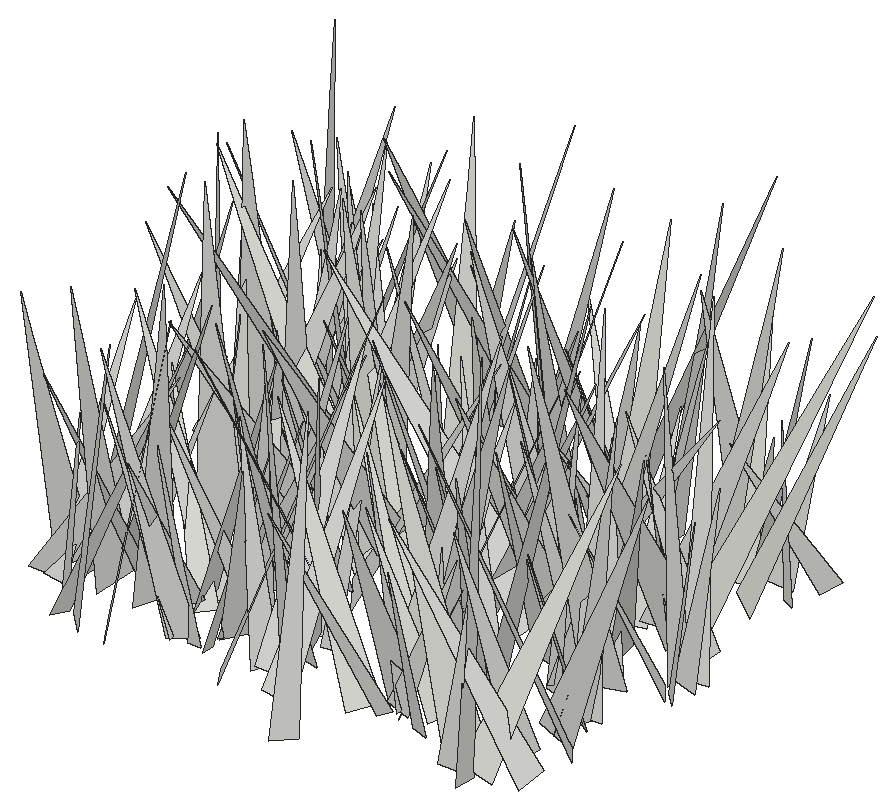
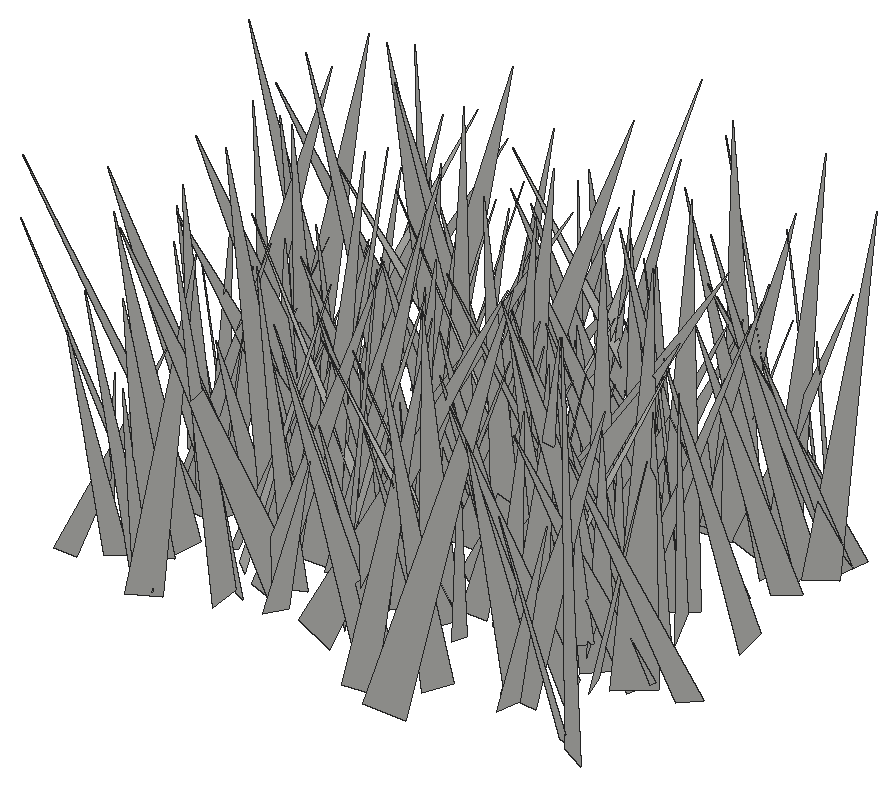
# SketchUp Ruby script. Lengths in inches.
U = 1.inch
M = Sketchup.active_model
def pt(a) = Geom::Point3d.new(a.map { |v| v * U })
def face(e, loops, mat)
  f = e.add_face(loops[0].map { |a| pt(a) })
  loops[1..].each { |l| e.add_face(l.map { |a| pt(a) }).erase! }
  f.material = f.back_material = mat if mat
  f
end
# faces: each face lists its corners as indices into pts; further lists are holes
def faces(e, pts, list, mat = nil) = list.each { |f| face(e, (f[0].is_a?(Array) ? f : [f]).map { |l| l.map { |i| pts[i] } }, mat) }
# xy, xz, yz: faces in a plane at the given z, y or x. An outline is a flat list of corners, or four numbers for a rectangle; further outlines are holes
def ring(l) = l.size == 4 ? [[l[0], l[1]], [l[2], l[1]], [l[2], l[3]], [l[0], l[3]]] : l.each_slice(2).to_a
def flat(e, list, mat, &to3) = list.each { |f| face(e, (f[0].is_a?(Array) ? f : [f]).map { |l| ring(l).map { |u, v| to3.(u, v) } }, mat) }
def xy(e, z, list, mat = nil) = flat(e, list, mat) { |x, y| [x, y, z] }
def xz(e, y, list, mat = nil) = flat(e, list, mat) { |x, z| [x, y, z] }
def yz(e, x, list, mat = nil) = flat(e, list, mat) { |y, z| [x, y, z] }
def lines(e, pts, list) = list.each { |a, b| e.add_line(pt(pts[a]), pt(pts[b])) }
# prism: a flat outline (further loops are holes) pulled along v
def prism(e, loops, v, mat = nil)
  f = face(e, loops, mat); d = Geom::Vector3d.new(v.map { |x| x * U })
  f.pushpull(f.normal.samedirection?(d) ? d.length : -d.length)
end
def box(e, o, s, mat = nil) = prism(e, [[o, [o[0] + s[0], o[1], o[2]], [o[0] + s[0], o[1] + s[1], o[2]], [o[0], o[1] + s[1], o[2]]]], [0, 0, s[2]], mat)
def at(x, y, z, deg = 0) = Geom::Transformation.translation(pt([x, y, z])) * Geom::Transformation.rotation(ORIGIN, Z_AXIS, deg.degrees)
def axes(o, x, y, z) = Geom::Transformation.new([*x, 0, *y, 0, *z, 0, *pt(o).to_a, 1])
def part(name) = M.definitions.add(name)
# library, detail: a bought-in or finely detailed component or shape, given as its bounding box
def library(name, o, s) = part(name).tap { |d| box(d.entities, o, s) }
def detail(e, o, s) = box(e.add_group.entities, o, s)
def put(e, d, t, mat = nil) = e.add_instance(d, t).tap { |i| i.material = mat if mat }
def group(e, t, mat = nil) = e.add_group.tap { |g| g.transformation = t; g.material = mat if mat }.entities
root = M.entities
c1 = part("fur_instance\#9")
p = [[0.8125,0,1.79],[0.67,-0.02,1.48],[0,-0.11,0],[0,0.11,0]]
faces(c1.entities,p,[[0,1,2,3]])
put(root,c1,axes([150.06,394.9,-27.1],[-5.67085,1.89535,1.35099],[1.57668,5.74544,-1.44226],[1.71219,0.98676,5.80265]))
put(root,c1,axes([155.92,397,-27.1],[0.94774,-3.5048,1.15841],[-3.67796,-0.79512,0.60341],[0.31324,1.26803,3.58018]))
put(root,c1,axes([140.08,397.19,-27.1],[6.22111,3.48137,1.76986],[3.77865,-6.20685,-1.07301],[-0.98698,-1.81924,7.04775]))
put(root,c1,axes([158.84,398.09,-27.1],[-5.67147,0.82087,0.04901],[0.80443,5.46726,1.5178],[-0.17066,-1.50898,5.5259]))
put(root,c1,axes([138.85,396.97,-27.1],[4.00395,3.96639,1.91354],[4.25291,-4.1539,-0.28869],[-1.14309,-1.56151,5.62855]))
put(root,c1,axes([153.53,398.33,-27.1],[-0.97443,-3.66118,0.75209],[-3.71136,1.03977,0.25308],[0.44234,0.6588,3.78017]))
put(root,c1,axes([142.61,398.41,-27.1],[0.82361,-5.861,1.93807],[-5.93962,-1.28507,-1.3621],[-1.68178,1.66825,5.75972]))
put(root,c1,axes([151.41,400.09,-27.1],[5.27025,-2.47106,0.85487],[-2.00329,-5.05203,-2.25305],[-1.68041,-1.72721,5.36707]))
put(root,c1,axes([157.63,399.32,-27.1],[-4.78026,1.17069,2.19317],[1.89155,4.79719,1.56216],[1.61324,-2.15588,4.66702]))
put(root,c1,axes([155.46,398.49,-27.1],[3.76435,-5.16952,3.38659],[-5.24976,-4.76711,-1.44149],[-3.26082,1.70703,6.23028]))
put(root,c1,axes([137.65,397.86,-27.1],[-2.04031,-2.94511,1.87891],[-3.25881,2.38849,0.20512],[1.25863,1.41005,3.57693]))
put(root,c1,axes([138.14,400.1,-27.1],[6.98441,-2.34407,2.00985],[-1.86712,-7.16517,-1.86827],[-2.45928,-1.21733,7.12645]))
put(root,c1,axes([151.6875,398.65,-27.1],[-1.12844,-4.06047,0.83548],[-3.60524,0.5338,-2.27512],[-2.04639,1.29864,3.54749]))
put(root,c1,axes([141.48,400.43,-27.1],[3.03189,-3.59681,0.02756],[-3.43565,-2.90654,-1.37057],[-1.06494,-0.8632,4.50011]))
put(root,c1,axes([157.08,396.49,-27.1],[-7.37531,-1.40171,2.74866],[-2.16749,7.42249,-2.03071],[2.19589,2.61858,7.22747]))
put(root,c1,axes([143.98,399.68,-27.1],[3.85722,-2.97975,0.1804],[-2.96484,-3.85827,-0.33622],[-0.3481,-0.15623,4.86251]))
put(root,c1,axes([142.22,398.5,-27.1],[-4.50006,-1.01814,0.39176],[-1.03948,4.50642,-0.22865],[0.331,0.31016,4.60813]))
put(root,c1,axes([147.51,401.94,-27.1],[-4.65731,-6.85842,0.0184],[-6.74044,4.58127,1.51895],[1.26677,-0.83835,8.14992]))
put(root,c1,axes([136.05,400.48,-27.1],[5.91516,-3.3432,1.65321],[-2.9566,-6.09276,-1.74243],[-2.27346,-0.77492,6.56735]))
put(root,c1,axes([143.23,398.31,-27.1],[0.75971,3.71481,1.88794],[3.89435,-1.31575,1.02184],[-1.48263,-1.55251,3.65142]))
put(root,c1,axes([146.2,398.67,-27.1],[-4.24357,2.27798,1.78244],[2.54082,4.44811,0.36434],[1.38223,-1.18292,4.80254]))
put(root,c1,axes([140.07,399.95,-27.1],[6.97183,-3.45055,1.53762],[-3.37643,-7.13932,-0.71191],[-1.69419,0.0288,7.74635]))
put(root,c1,axes([148.16,397.59,-27.1],[-6.10428,-1.79449,1.71008],[-2.20054,6.01533,-1.54278],[1.14113,2.0006,6.1727]))
put(root,c1,axes([139.66,400.42,-27.1],[-1.20375,-5.21342,0.24756],[-5.17288,1.15789,-0.76855],[-0.69453,0.4118,5.2951]))
put(root,c1,axes([151.89,399.15,-27.1],[0.78956,-4.05986,1.16414],[-3.93825,-0.27989,1.69498],[1.52574,1.37851,3.77266]))
put(root,c1,axes([150.81,398.53,-27.1],[-4.45803,3.98436,0.74293],[4.03358,4.25341,1.39275],[-0.39655,-1.52789,5.81458]))
put(root,c1,axes([137.97,397.15,-27.1],[5.78446,0.51407,0.77192],[0.25637,-5.57234,1.78981],[-0.89129,1.73346,5.52457]))
put(root,c1,axes([147.09,399.9,-27.1],[-2.90211,-6.23156,1.67253],[-6.44447,2.71044,-1.08359],[-0.31368,1.96803,6.78825]))
put(root,c1,axes([156.99,397.26,-27.1],[0.07577,6.70614,0.84141],[6.48392,0.16538,-1.90197],[1.90764,-0.82847,6.43122]))
put(root,c1,axes([153.46,399.5625,-27.1],[-3.79672,1.89832,0.59417],[1.98792,3.66583,0.99077],[0.06937,-1.15319,4.1276]))
put(root,c1,axes([147.94,397.125,-27.1],[0.187,6.43803,0.46404],[6.40843,-0.12967,-0.78342],[0.77175,-0.48321,6.39292]))
put(root,c1,axes([135.7,399.11,-27.1],[4.06898,-3.86093,0.67624],[-3.71406,-3.48612,2.44405],[1.25293,2.20473,5.04877]))
put(root,c1,axes([158.81,400.48,-27.1],[-5.4011,-4.4458,0.12135],[-4.40164,5.31613,-1.14717],[-0.63674,0.96192,6.9008]))
put(root,c1,axes([143.81,398.35,-27.1],[3.84083,1.33111,0.88578],[1.09907,-3.87194,1.0529],[-1.16125,0.73803,3.92622]))
put(root,c1,axes([152,399.375,-27.1],[-4.7779,-0.84592,1.0787],[-0.97294,4.84801,-0.50762],[0.9657,0.69908,4.82558]))
put(root,c1,axes([145.41,397.03,-27.1],[6.47525,4.61232,0.40047],[4.47579,-6.41261,1.48613],[-1.18373,0.98374,7.80985]))
put(root,c1,axes([152.64,400.59,-27.1],[1.6475,-3.20979,0.84583],[-3.31321,-1.64761,0.20101],[-0.20196,0.8456,3.6023]))
put(root,c1,axes([157.54,401.13,-27.1],[1.03631,-6.95808,1.71035],[-6.57848,-0.23906,3.0134],[2.83968,1.98547,6.35675]))
put(root,c1,axes([146.55,401.06,-27.1],[5.52429,1.58059,2.16664],[1.98524,-5.74559,-0.8703],[-1.80317,-1.48335,5.67966]))
put(root,c1,axes([137.67,401.22,-27.1],[7.30646,0.41261,0.41525],[0.46932,-7.23653,-1.06747],[-0.34987,-1.09065,7.23983]))
put(root,c1,axes([143.98,401.01,-27.1],[-0.35504,-4.51922,1.36303],[-4.31721,-0.2418,-1.92625],[-1.90863,1.3876,4.10353]))
put(root,c1,axes([146.66,398.4375,-27.1],[-1.23708,6.4323,0.84499],[6.38548,1.35924,-0.99849],[1.14637,-0.62994,6.47363]))
put(root,c1,axes([141.63,400.9,-27.1],[5.98361,0.11352,0.76596],[0.13466,-6.02993,-0.15823],[-0.76252,-0.17402,5.9826]))
put(root,c1,axes([136.29,398.97,-27.1],[0.97806,5.36378,0.25201],[5.36787,-0.98334,0.09641],[-0.14015,-0.23057,5.45137]))
put(root,c1,axes([143.35,401.77,-27.1],[4.53528,-3.04969,1.17101],[-3.07507,-4.66168,-0.23091],[-1.10265,0.45689,5.46041]))
put(root,c1,axes([149.2,400.67,-27.1],[-4.27231,-1.94809,0.06255],[-1.87913,4.07681,-1.37844],[-0.51754,1.27912,4.48861]))
put(root,c1,axes([157.16,401.75,-27.1],[4.10425,1.09153,0.3293],[1.14011,-3.92312,-1.20584],[0.00571,-1.24998,4.07214]))
put(root,c1,axes([151.17,400.07,-27.1],[1.96643,7.28816,1.86053],[7.47956,-1.69089,-1.28167],[0.79683,-2.11408,7.43918]))
put(root,c1,axes([143.74,399.33,-27.1],[3.9731,1.20771,1.01378],[0.70264,-3.81635,1.79266],[-1.41159,1.49959,3.74573]))
put(root,c1,axes([151.63,400.76,-27.1],[-3.45745,4.3845,0.64107],[4.38114,3.2607,1.32749],[-0.66366,-1.31634,5.42361]))
put(root,c1,axes([152.15,403.32,-27.1],[-0.85203,-5.57664,0.61964],[-5.3803,0.98986,1.51043],[1.59225,0.36067,5.43539]))
put(root,c1,axes([150.91,402.38,-27.1],[6.79044,-4.4332,0.71146],[-4.48312,-6.76549,0.63187],[-0.24718,0.91888,8.0848]))
put(root,c1,axes([141.97,400.49,-27.1],[-2.66965,3.73747,0.14274],[3.69986,2.61324,0.77338],[-0.54785,-0.56423,4.52743]))
put(root,c1,axes([141.83,401.4,-27.1],[-5.56985,2.38046,0.65327],[2.45077,5.52546,0.76123],[0.29505,-0.95874,6.00918]))
put(root,c1,axes([152.17,399.02,-27.1],[5.76242,3.50846,0.12226],[3.39302,-5.62636,1.53663],[-0.90093,1.2508,6.56914]))
put(root,c1,axes([157.83,402.36,-27.1],[-2.17535,-3.01047,0.60266],[-3.06621,2.16789,-0.23847],[0.15643,0.62897,3.70651]))
put(root,c1,axes([152.35,403.72,-27.1],[-3.97091,-3.72473,0.66515],[-3.58252,4.01146,1.07602],[1.21718,-0.34456,5.33703]))
put(root,c1,axes([136.98,400.17,-27.1],[7.21368,2.51232,2.17903],[2.05011,-7.45745,1.81123],[-2.61859,1.08246,7.42081]))
put(root,c1,axes([146.46,401.7,-27.1],[-0.50007,3.75556,1.02909],[3.87876,0.38868,0.46638],[-0.34425,-1.07612,3.75989]))
put(root,c1,axes([147.2,406.47,-27.1],[4.97759,-6.71856,0.2944],[-6.18791,-4.7191,-3.07278],[-2.63353,-1.61035,7.77647]))
put(root,c1,axes([142.9,400.64,-27.1],[1.96135,3.70682,0.36248],[3.45553,-1.96392,1.38604],[-1.38968,0.34826,3.95807]))
put(root,c1,axes([149.18,404.94,-27.1],[7.15666,-2.1147,0.99823],[-1.83229,-7.06792,-1.83669],[-1.45298,-1.50292,7.233]))
put(root,c1,axes([157.6875,402.47,-27.1],[5.90361,-0.69248,2.28384],[-0.937,-6.27702,0.51884],[-2.19488,0.81708,5.9214]))
put(root,c1,axes([150.68,405.24,-27.1],[-1.15105,-5.30671,0.17],[-5.09537,1.15297,1.49093],[1.49242,-0.15644,5.22142]))
put(root,c1,axes([142.31,403.23,-27.1],[-3.28529,-1.60429,1.12724],[-1.66632,3.44368,0.04462],[1.03333,0.45264,3.6558]))
put(root,c1,axes([156.66,405.05,-27.1],[1.61042,-7.88282,1.5376],[-7.97737,-1.75156,-0.62458],[-0.92985,1.37466,8.02136]))
put(root,c1,axes([142.35,402.32,-27.1],[5.41003,-2.25588,0.78895],[-2.38957,-5.13634,1.69936],[-0.03699,1.87321,5.60977]))
put(root,c1,axes([136.34,402.07,-27.1],[-0.72846,5.64896,1.65026],[5.62241,1.15927,-1.48642],[1.73859,-1.38206,5.49837]))
put(root,c1,axes([153.78,405.26,-27.1],[-0.77388,-5.77446,0.46112],[-5.72229,0.83441,0.84559],[0.90132,0.33953,5.76439]))
put(root,c1,axes([153.49,402.61,-27.1],[8.05424,1.38868,1.7961],[1.29513,-8.24767,0.56905],[-1.86468,0.26973,8.15325]))
put(root,c1,axes([147.1875,401.08,-27.1],[1.91748,5.33638,0.31642],[5.10909,-1.9283,1.55969],[-1.57297,0.24194,5.4517]))
put(root,c1,axes([150.89,405,-27.1],[-5.52316,-3.7636,0.965],[-3.71814,5.60658,0.58551],[1.12752,0.05244,6.65787]))
put(root,c1,axes([137.57,402.83,-27.1],[2.54826,3.20038,0.28055],[3.20908,-2.5526,-0.02947],[-0.15164,-0.23787,4.09087]))
put(root,c1,axes([138.67,405.51,-27.1],[5.1556,-5.75467,2.21602],[-5.90961,-5.43588,-0.36737],[-1.76168,1.39363,7.71761]))
put(root,c1,axes([145.36,404.65,-27.1],[5.77692,4.11347,0.10405],[3.90568,-5.42514,-2.37018],[1.29504,-1.98782,6.68399]))
put(root,c1,axes([158.59,406.08,-27.1],[-3.47143,-2.84551,0.09651],[-2.81271,3.45107,0.57956],[0.4415,-0.38766,4.45106]))
put(root,c1,axes([155.74,407.03,-27.1],[6.93671,-0.62868,0.23505],[-0.51232,-6.5363,-2.3628],[-0.4336,-2.33453,6.55213]))
put(root,c1,axes([157.57,402.875,-27.1],[1.24745,7.40868,1.63783],[7.39275,-1.56046,1.42803],[-1.70827,-1.34297,7.376]))
put(root,c1,axes([155.36,405.58,-27.1],[0.47741,-4.86513,1.33169],[-4.92648,-0.73691,-0.92606],[-1.08291,1.20759,4.79999]))
put(root,c1,axes([144.97,404.88,-27.1],[0.7235,3.49331,2.20248],[3.65755,-1.58024,1.30491],[-1.91742,-1.69623,3.32022]))
put(root,c1,axes([142.81,403.1,-27.1],[5.29795,0.17393,1.896],[-0.4687,-5.31448,1.7972],[-1.84537,1.84915,4.98684]))
put(root,c1,axes([141.83,407.66,-27.1],[2.44843,-5.51273,0.60157],[-4.8536,-2.44839,-2.68234],[-2.6823,-0.60174,5.40279]))
put(root,c1,axes([138.97,404.72,-27.1],[5.52113,3.74347,2.2115],[4.00437,-5.77059,-0.2291],[-1.6939,-1.44011,6.66663]))
put(root,c1,axes([155.43,403.62,-27.1],[2.35955,4.93164,1.36493],[4.86886,-2.62618,1.07189],[-1.57426,-0.73054,5.36093]))
put(root,c1,axes([152.09,408.16,-27.1],[4.15216,-5.25606,0.30062],[-4.95254,-4.0295,-2.04756],[-1.78575,-1.04593,6.37763]))
put(root,c1,axes([151.65,404.47,-27.1],[-4.9618,2.41645,1.1014],[2.44275,5.06865,-0.11597],[1.04177,-0.37582,5.51772]))
put(root,c1,axes([149.36,404.625,-27.1],[-0.86303,4.80618,1.97762],[4.83833,1.47497,-1.47315],[1.8976,-1.57489,4.65553]))
put(root,c1,axes([155.25,405.69,-27.1],[-0.48209,-3.49328,1.24378],[-3.69826,0.54426,0.09516],[0.26993,1.21786,3.5251]))
put(root,c1,axes([157.15,409.34,-27.1],[4.52461,-6.7861,0.00105],[-6.53347,-4.35651,-2.20405],[-1.83437,-1.22185,7.85273]))
put(root,c1,axes([149.17,404.12,-27.1],[-2.13966,5.92839,0.3544],[5.56639,1.87053,2.31645],[-2.07043,-1.09766,5.86157]))
put(root,c1,axes([152.4375,408.11,-27.1],[-3.66849,-5.82093,1.22872],[-5.44278,3.86666,2.06783],[2.40191,-0.1285,6.56241]))
put(root,c1,axes([151.82,407.34,-27.1],[-7.78216,2.50032,0.23977],[2.4235,7.26917,2.85602],[-0.66011,-2.78901,7.65877]))
put(root,c1,axes([139.53,407.34,-27.1],[-6.5147,0.26004,1.16019],[0.55336,6.38259,1.67669],[1.05235,-1.74639,6.3006]))
put(root,c1,axes([156.18,405.84,-27.1],[-2.69115,3.5868,1.84623],[3.86426,2.92918,-0.05799],[1.15809,-1.43902,4.48375]))
put(root,c1,axes([159.03,405.85,-27.1],[-2.22453,-2.28888,1.93607],[-2.6411,2.63697,0.08289],[1.41842,1.32035,3.19071]))
put(root,c1,axes([144.74,407.35,-27.1],[4.88048,-6.02987,2.56967],[-6.14977,-5.32095,-0.80587],[-2.26779,1.4525,7.7155]))
put(root,c1,axes([158.85,406.87,-27.1],[0.22976,-4.49295,1.68417],[-4.67204,0.17468,1.10336],[1.09322,1.69077,4.36142]))
put(root,c1,axes([144.38,408.95,-27.1],[-2.23996,-8.03771,0.28468],[-7.44594,1.96073,-3.22749],[-3.04036,1.11981,7.69451]))
put(root,c1,axes([135.1,405.7,-27.1],[6.05583,0.88682,1.38397],[0.67013,-6.15634,1.01257],[-1.50092,0.82941,6.03608]))
put(root,c1,axes([155.43,404.32,-27.1],[7.73551,0.03019,2.73159],[-1.01366,-7.58581,2.95441],[-2.53672,3.12332,7.14916]))
put(root,c1,axes([144.4375,407.9,-27.1],[0.04247,-7.07988,2.41623],[-7.48051,-0.06275,-0.05238],[-0.06984,2.41579,7.07981]))
put(root,c1,axes([149.96,406.57,-27.1],[5.54197,-0.978,0.47716],[-1.05474,-5.437,1.10644],[-0.26776,1.17482,5.51777]))
put(root,c1,axes([139.78,408.5625,-27.1],[6.66168,-2.88093,2.18206],[-2.80757,-7.00677,-0.67958],[-2.27567,0.211,7.22605]))
put(root,c1,axes([158.44,407.0625,-27.1],[-5.81537,-0.03657,1.70774],[-0.23888,6.01751,-0.6846],[1.69135,0.72416,5.77505]))
put(root,c1,axes([145.93,408.32,-27.1],[-2.3451,-4.39084,0.71964],[-4.31416,2.04482,-1.58228],[-1.08875,1.35503,4.71968]))
put(root,c1,axes([144.76,406.84,-27.1],[-4.02573,7.19257,0.41274],[6.48293,3.4104,3.80141],[-3.14246,-2.17854,7.31361]))
put(root,c1,axes([157.27,408.23,-27.1],[-3.81411,-2.18756,1.38745],[-2.30966,3.98998,-0.05835],[1.17299,0.74331,4.39652]))
put(root,c1,axes([151.97,407.66,-27.1],[4.55,-4.60588,0.41001],[-4.16176,-3.82822,3.1795],[2.01545,2.49305,5.6398]))
put(root,c1,axes([142.47,405.12,-27.1],[2.76635,7.35948,0.05567],[7.35952,-2.76581,-0.07342],[0.04914,-0.07794,7.86188]))
put(root,c1,axes([143.23,409.17,-27.1],[0.67729,-7.55263,2.0847],[-7.70125,-0.25666,1.57216],[1.44182,2.17688,7.41817]))
put(root,c1,axes([158.24,408.97,-27.1],[-5.1344,0.67452,1.09766],[0.89094,5.11676,1.02317],[0.93062,-1.17714,5.07643]))
put(root,c1,axes([144.15,410.25,-27.1],[0.26999,-5.16111,0.17986],[-5.16087,-0.27616,-0.17741],[-0.18667,0.17024,5.16512]))
put(root,c1,axes([137.7,406.43,-27.1],[-6.50203,-1.48304,1.94789],[-2.15091,6.10063,-2.53495],[1.1693,2.97539,6.16846]))
put(root,c1,axes([138.15,407.15,-27.1],[0.38602,5.6901,1.15392],[5.67114,-0.61727,1.14668],[-1.24374,-1.04858,5.58671]))
put(root,c1,axes([137.91,409.85,-27.1],[3.24769,-2.54753,0.32293],[-2.51539,-3.26077,-0.4265],[-0.51676,-0.13836,4.10555]))
put(root,c1,axes([150.83,410.82,-27.1],[-0.69616,-7.71222,1.47846],[-7.81205,0.83092,0.65597],[0.79755,1.40715,7.71575]))
put(root,c1,axes([152.71,411.24,-27.1],[3.43107,-2.8474,0.0502],[-2.64084,-3.2106,-1.6126],[-1.06592,-1.21113,4.15686]))
put(root,c1,axes([138.87,407.95,-27.1],[-2.71022,2.78687,0.60598],[2.7235,2.77712,-0.59105],[0.8464,-0.01233,3.84222]))
put(root,c1,axes([153.89,411.8,-27.1],[-4.54437,-2.07997,0.71062],[-1.49312,4.11891,2.50752],[1.61302,-2.04715,4.32318]))
put(root,c1,axes([149.75,410.67,-27.1],[-6.14349,2.42883,3.06477],[3.31416,6.26335,1.67969],[2.07568,-2.81172,6.38908]))
put(root,c1,axes([151.89,409.95,-27.1],[4.55769,0.07164,0.01251],[0.0727,-4.46545,-0.91231],[0.00209,-0.91239,4.46602]))
put(root,c1,axes([158.87,407.35,-27.1],[0.5538,7.06628,1.29605],[7.05626,-0.7792,1.23321],[-1.34954,-1.17443,6.97985]))
put(root,c1,axes([148.31,408.86,-27.1],[4.95013,-1.23925,0.4471],[-1.29852,-4.88303,0.8422],[-0.22245,0.9272,5.03291]))
put(root,c1,axes([147.76,411.75,-27.1],[0.04578,-6.29285,0.19538],[-6.21134,-0.07706,-1.02644],[-1.02831,0.18529,6.20874]))
put(root,c1,axes([136.24,410.95,-27.1],[5.79688,-5.3049,1.7816],[-5.31494,-6.02201,-0.63769],[-1.75142,0.71643,7.83193]))
put(root,c1,axes([148.92,409.12,-27.1],[6.16739,3.42449,0.19717],[3.4017,-6.05394,-1.25736],[0.441,-1.19388,6.94138]))
put(root,c1,axes([148.3,408.59,-27.1],[2.54415,2.86578,1.34064],[2.68524,-2.86561,1.02977],[-1.67317,-0.2414,3.6912]))
put(root,c1,axes([147.15,409.23,-27.1],[-5.93557,-1.05009,0.32847],[-1.08922,5.86272,-0.94003],[0.15548,0.98355,5.95399]))
put(root,c1,axes([146.39,411.46,-27.1],[5.5268,-1.95543,1.04999],[-1.67194,-5.52102,-1.48142],[-1.45972,-1.07995,5.67227]))
put(root,c1,axes([137.53,408.62,-27.1],[-2.26569,5.88907,2.62757],[5.5866,3.18358,-2.31806],[3.22106,-1.37923,5.86866]))
put(root,c1,axes([141.54,410.82,-27.1],[-5.94217,-4.1756,0.21971],[-4.13273,5.80684,-1.41225],[-0.63601,1.27993,7.12394]))
put(root,c1,axes([155.44,409.77,-27.1],[4.70932,-5.02611,1.74089],[-5.27526,-4.11549,2.38842],[0.68127,2.87596,6.46026]))
put(root,c1,axes([153.48,409.53,-27.1],[-0.77106,7.66776,2.67234],[8.04873,1.0768,-0.76736],[1.07416,-2.56446,7.66813]))
put(root,c1,axes([142.625,408.93,-27.1],[-6.42625,-2.81034,1.42452],[-3.14557,5.90814,-2.53441],[0.18076,2.90169,6.53999]))
put(root,c1,axes([154.64,409.25,-27.1],[-1.99149,3.68652,0.84504],[3.6319,2.13053,-0.73532],[1.05538,-0.37542,4.12502]))
put(root,c1,axes([138.19,410.44,-27.1],[-3.99726,2.72851,1.81883],[2.89094,4.28575,-0.07581],[1.5477,-0.9584,4.83912]))
put(root,c1,axes([152.8,412.71,-27.1],[-3.72414,-4.2026,0.59605],[-4.10843,3.76818,0.89886],[1.06672,-0.15915,5.54285]))
put(root,c1,axes([138.09,410.7,-27.1],[3.39124,-4.48702,2.29298],[-4.9912,-3.37077,0.78574],[-0.69206,2.32297,5.56924]))
put(root,c1,axes([145.99,409.12,-27.1],[3.94824,4.29759,0.4959],[4.2386,-3.97723,0.72087],[-0.86569,0.12707,5.79122]))
put(root,c1,axes([147.875,411.47,-27.1],[-2.80028,2.24736,2.49663],[2.73085,3.4158,-0.01176],[1.95607,-1.55147,3.59055]))
put(root,c1,axes([141.38,410.47,-27.1],[-0.70822,-5.57958,3.0516],[-6.3293,0.31925,-0.88519],[-0.61961,3.1164,5.55425]))
put(root,c1,axes([149.0625,412.41,-27.1],[-4.24041,-4.62675,0.86788],[-4.65391,4.29598,0.16351],[0.70788,0.52807,6.27385]))
put(root,c1,axes([138.03,409.42,-27.1],[7.54644,-1.30772,2.23251],[-1.88035,-7.50036,1.96263],[-1.77721,2.38276,7.40318]))
put(root,c1,axes([143.09,409.68,-27.1],[-5.60196,1.71083,0.59088],[1.59688,5.57635,-1.00614],[0.85208,0.79713,5.77032]))
put(root,c1,axes([140.47,409.98,-27.1],[0.3651,6.79595,1.75212],[7.01816,-0.34958,-0.10649],[0.01583,-1.75528,6.80491]))
put(root,c1,axes([141.18,410.77,-27.1],[4.31663,-3.25233,1.38409],[-3.53279,-4.03972,1.52536],[-0.11299,2.05661,5.185]))
put(root,c1,axes([137.58,411.6,-27.1],[-4.67685,-1.64881,1.07356],[-1.71505,4.77313,-0.14071],[0.96421,0.49258,4.95698]))
put(root,c1,axes([140.96,411.3,-27.1],[-6.02179,2.8816,2.13168],[3.11245,6.27078,0.31555],[1.77772,-1.21792,6.66828]))
put(root,c1,axes([140.3125,411.93,-27.1],[5.34451,-3.5502,0.35957],[-3.55754,-5.25077,1.03462],[0.27778,1.05952,6.33224]))
put(root,c1,axes([143.46,411.95,-27.1],[3.51099,-0.42801,1.09439],[-0.295,-3.65871,-0.48452],[-1.13748,-0.37227,3.50364]))
put(root,c1,axes([136.15,410.64,-27.1],[3.23121,-4.00646,1.7311],[-4.24322,-2.37965,2.41277],[1.02152,2.78831,4.54653]))
put(root,c1,axes([156.83,409.81,-27.1],[0.48963,4.22721,0.04806],[3.94805,-0.47454,1.51627],[-1.51146,0.12987,3.97618]))
put(root,c1,axes([138.74,410.6875,-27.1],[-2.41477,3.3901,0.55663],[3.41153,2.44646,-0.10002],[0.40504,-0.3947,4.161]))
put(root,c1,axes([134.17,410.35,-27.1],[-0.28996,5.60424,1.15409],[5.32871,0.68543,-1.98963],[2.08431,-0.97272,5.24719]))
put(root,c1,axes([150.3,412.79,-27.1],[-0.32261,-5.78503,1.74562],[-5.69921,0.87225,1.8374],[2.00818,1.5461,5.49497]))
put(root,c1,axes([150.92,413.74,-27.1],[-1.61608,-6.86234,1.14057],[-6.89566,1.42577,-1.19223],[-0.91789,1.37106,6.94853]))
put(root,c1,axes([156.31,410.68,-27.1],[3.48936,7.09192,0.65775],[6.9322,-3.21357,-2.12629],[1.63479,-1.51038,7.61247]))
put(root,c1,axes([147.73,414.92,-27.1],[-1.57704,-7.74459,0.50786],[-7.45096,1.36569,-2.31124],[-2.17253,0.93802,7.55804]))
put(root,c1,axes([144.63,411.64,-27.1],[-6.2785,3.87073,1.88034],[3.7817,6.55006,-0.85632],[2.05354,-0.22787,7.32591]))
put(root,c1,axes([147.68,413.37,-27.1],[-5.07554,-4.81191,2.50581],[-5.17107,5.32884,-0.24106],[1.64121,1.90882,6.98981]))
put(root,c1,axes([138.97,414.16,-27.1],[1.01091,-5.94061,2.30759],[-6.04054,-1.63799,-1.57056],[-2.03168,1.91413,5.81775]))
put(root,c1,axes([156.77,412.875,-27.1],[3.72746,5.46093,0.78491],[5.42353,-3.45332,-1.72965],[1.01153,-1.60767,6.38153]))
put(root,c1,axes([144.35,412.63,-27.1],[4.3038,1.80689,1.01933],[1.67441,-4.41138,0.75005],[-1.22483,0.31842,4.60705]))
put(root,c1,axes([144.78,410.26,-27.1],[5.37795,5.75,0.47067],[5.40496,-5.24661,2.33794],[-2.01755,1.27162,7.51791]))
put(root,c1,axes([158.48,415.77,-27.1],[2.70067,-3.13661,0.88183],[-2.51329,-2.73437,-2.02883],[-2.07348,-0.77102,3.60774]))
put(root,c1,axes([146.38,413.11,-27.1],[5.52496,2.9641,0.73245],[3.00682,-5.54515,-0.24054],[-0.53047,-0.55942,6.26523]))
put(root,c1,axes([155.25,413.08,-27.1],[6.61649,-1.70465,2.3436],[-2.13195,-6.81989,1.0584],[-1.96294,1.66119,6.75008]))
put(root,c1,axes([145.32,414.11,-27.1],[4.26673,-0.51352,0.23406],[-0.5171,-4.27238,0.05285],[-0.22604,0.08052,4.29719]))
put(root,c1,axes([137.9,412.45,-27.1],[6.18202,1.83786,0.77531],[1.68935,-6.16651,1.14736],[-1.06062,0.8903,6.34654]))
put(root,c1,axes([151.6,414.41,-27.1],[3.4231,3.63538,1.50249],[3.93251,-3.11512,-1.42212],[0.09387,-2.06666,4.78656]))
put(root,c1,axes([157.96,413.94,-27.1],[1.56672,2.93333,1.48069],[3.11219,-1.85095,0.37383],[-1.05412,-1.105,3.30444]))
put(root,c1,axes([143.98,417.09,-27.1],[-0.13701,-6.93499,0.01519],[-6.899,0.13785,0.70555],[0.70571,0.00117,6.90036]))
put(root,c1,axes([142.22,417.8,-27.1],[1.01288,-8.11783,0.06805],[-8.08119,-1.01477,-0.77093],[-0.77341,-0.02823,8.14437]))
put(root,c1,axes([141.82,415.21,-27.1],[5.79925,-1.98106,0.58125],[-1.98372,-5.82701,-0.06806],[-0.57211,0.1232,6.12791]))
put(root,c1,axes([139.27,413.59,-27.1],[4.10356,-2.98524,2.70877],[-3.77942,-4.1935,1.10399],[-1.40181,2.56732,4.95298]))
put(root,c1,axes([154.3,416.47,-27.1],[4.71186,-4.25626,1.34995],[-4.06485,-4.9009,-1.26409],[-1.848,-0.07223,6.22249]))
put(root,c1,axes([156.91,414.79,-27.1],[-0.57371,3.97778,1.97621],[4.19128,1.14438,-1.08668],[1.47014,-1.71025,3.86924]))
put(root,c1,axes([155.93,414.72,-27.1],[5.31059,0.52385,1.16283],[0.52648,-5.43598,0.04446],[-1.16164,-0.06886,5.33618]))
put(root,c1,axes([155.65,414.03,-27.1],[-2.00411,5.21831,1.67163],[5.38658,2.20263,-0.41796],[1.00489,-1.39973,5.57427]))
put(root,c1,axes([150.6,413.05,-27.1],[8.13769,0.92636,1.08085],[0.65484,-8.00564,1.93114],[-1.26395,1.81658,7.95932]))
put(root,c1,axes([151.89,414.79,-27.1],[7.00703,0.38351,2.14023],[0.30488,-7.32356,0.31416],[-2.15283,0.21111,7.01048]))
put(root,c1,axes([139.01,414.7,-27.1],[-4.50468,1.1443,0.55643],[1.12699,4.53841,-0.20945],[0.5907,0.0676,4.64302]))
put(root,c1,axes([154.46,416.3125,-27.1],[0.84418,-3.62493,0.18375],[-3.45271,-0.74384,1.18829],[1.11924,0.43944,3.52714]))
put(root,c1,axes([149.88,414.45,-27.1],[-3.84574,2.31871,0.01808],[2.31862,3.84577,-0.02193],[0.02681,0.00945,4.49062]))
put(root,c1,axes([145.96,414.17,-27.1],[6.16496,0.12051,1.82007],[-0.27856,-6.27765,1.3592],[-1.80266,1.38221,6.01447]))
put(root,c1,axes([134.89,416.17,-27.1],[4.42565,6.01002,3.52258],[6.87552,-4.43985,-1.06317],[-1.12079,-3.50468,7.38759]))
put(root,c1,axes([135.84,415.45,-27.1],[2.6257,3.60497,0.95618],[3.72031,-2.44904,-0.98281],[0.26337,-1.34567,4.35019]))
